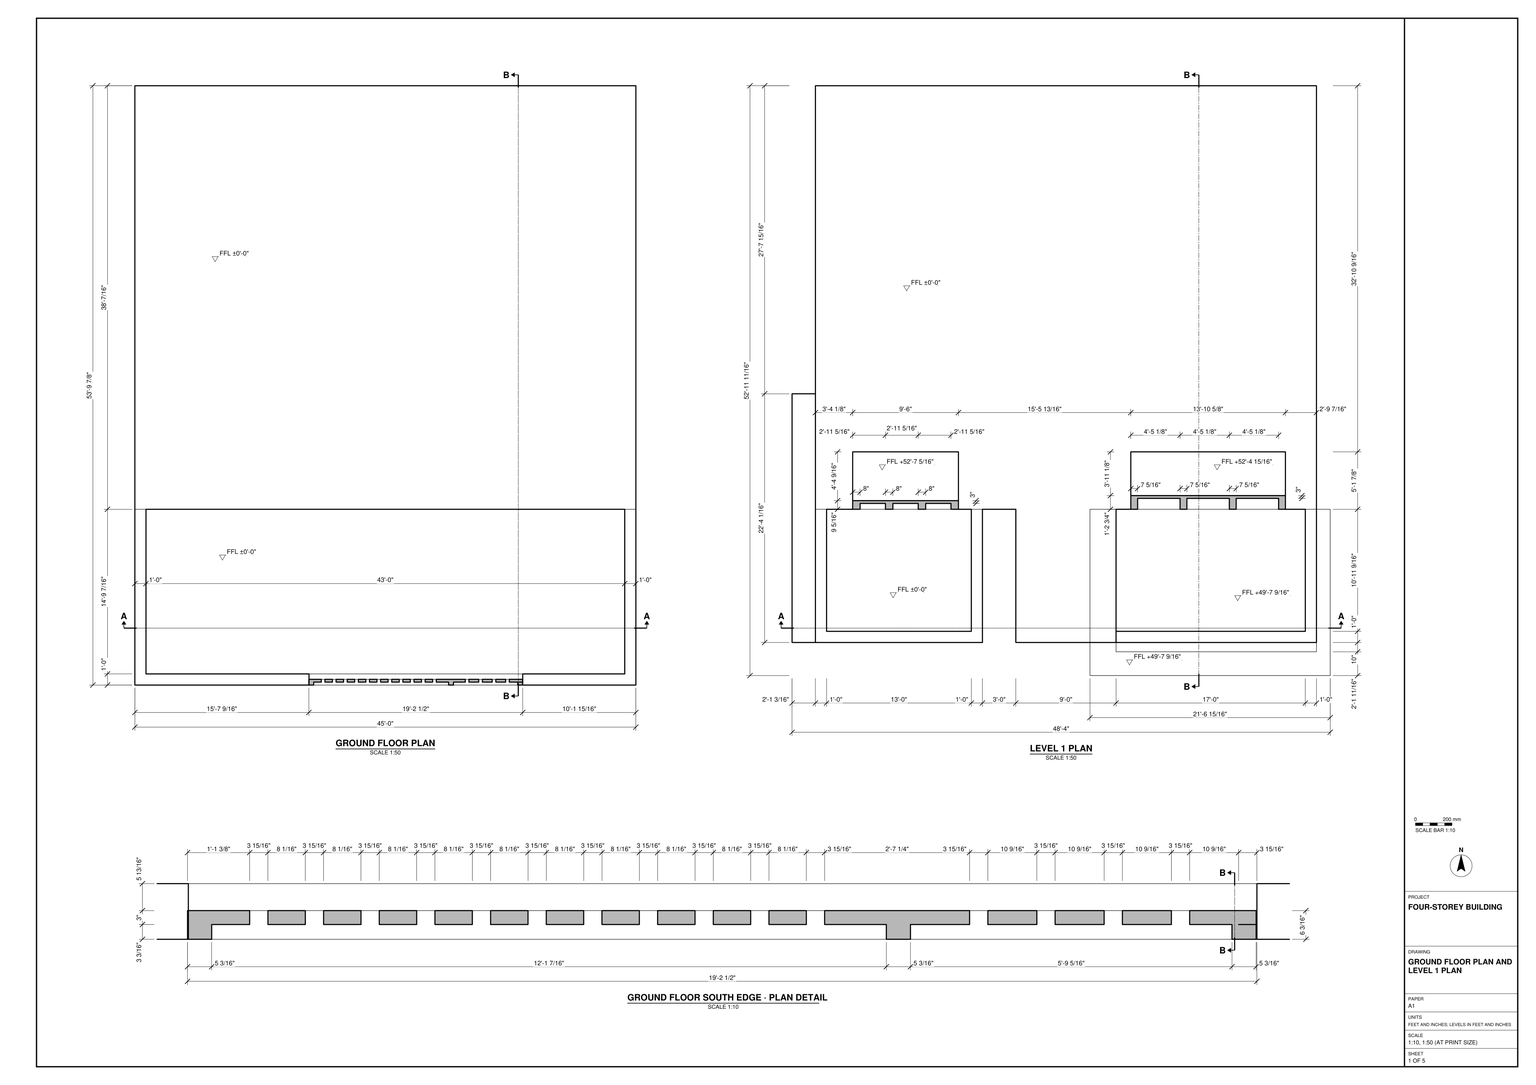
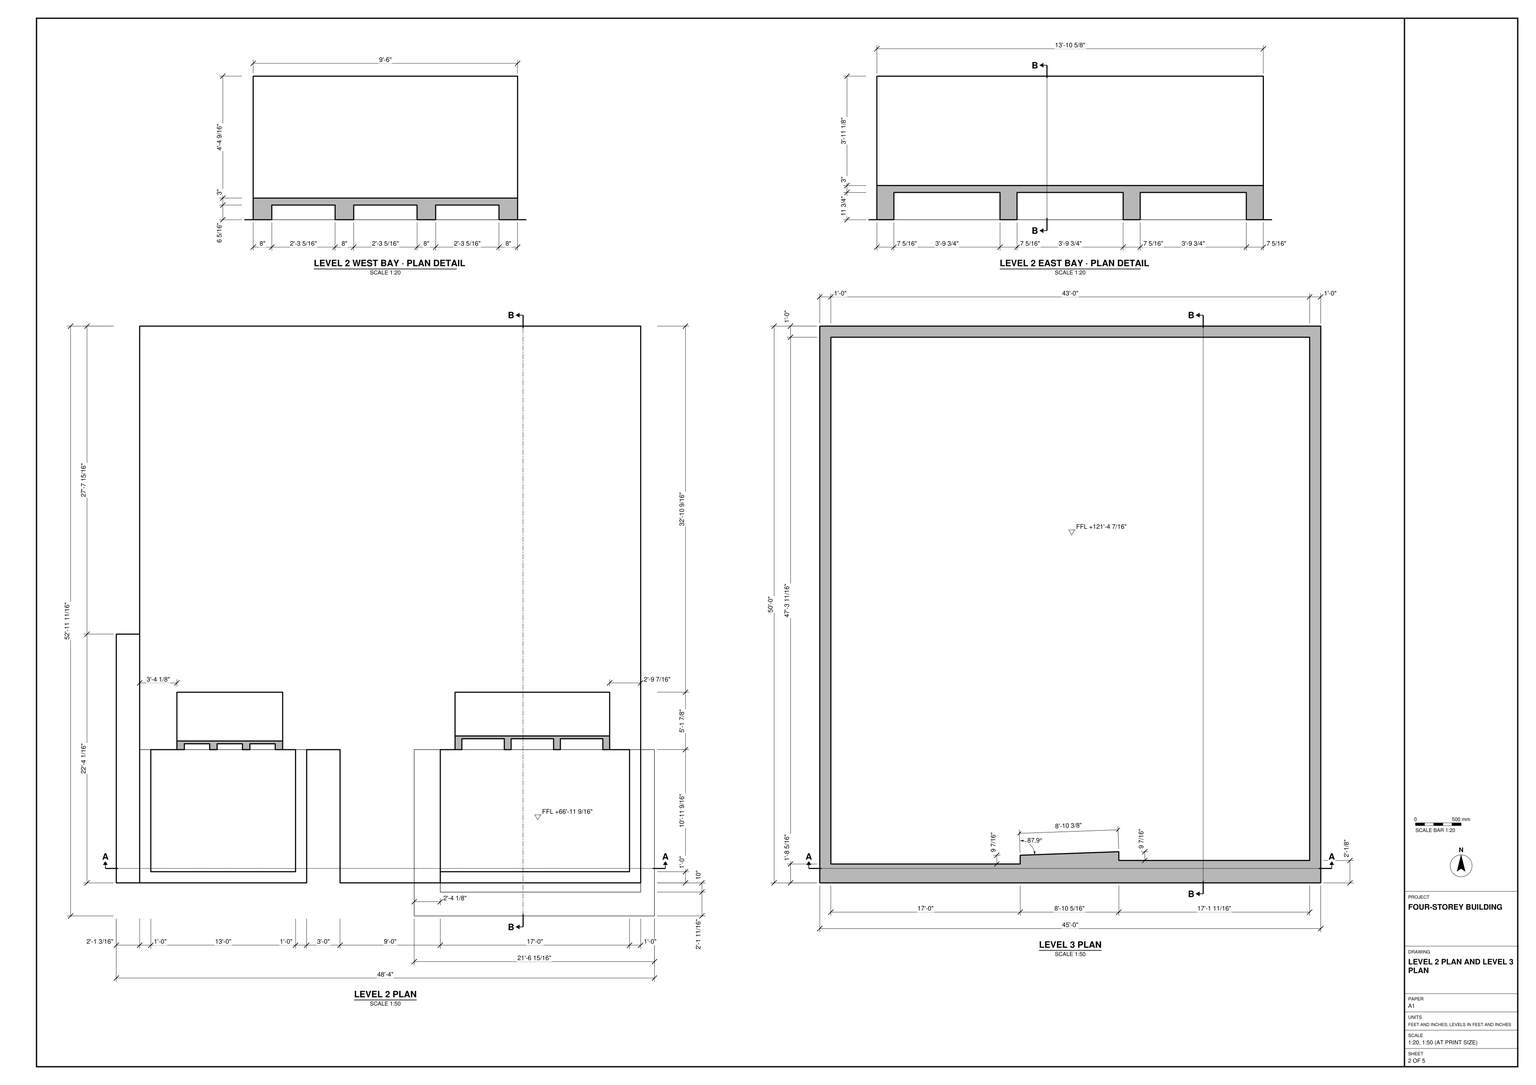
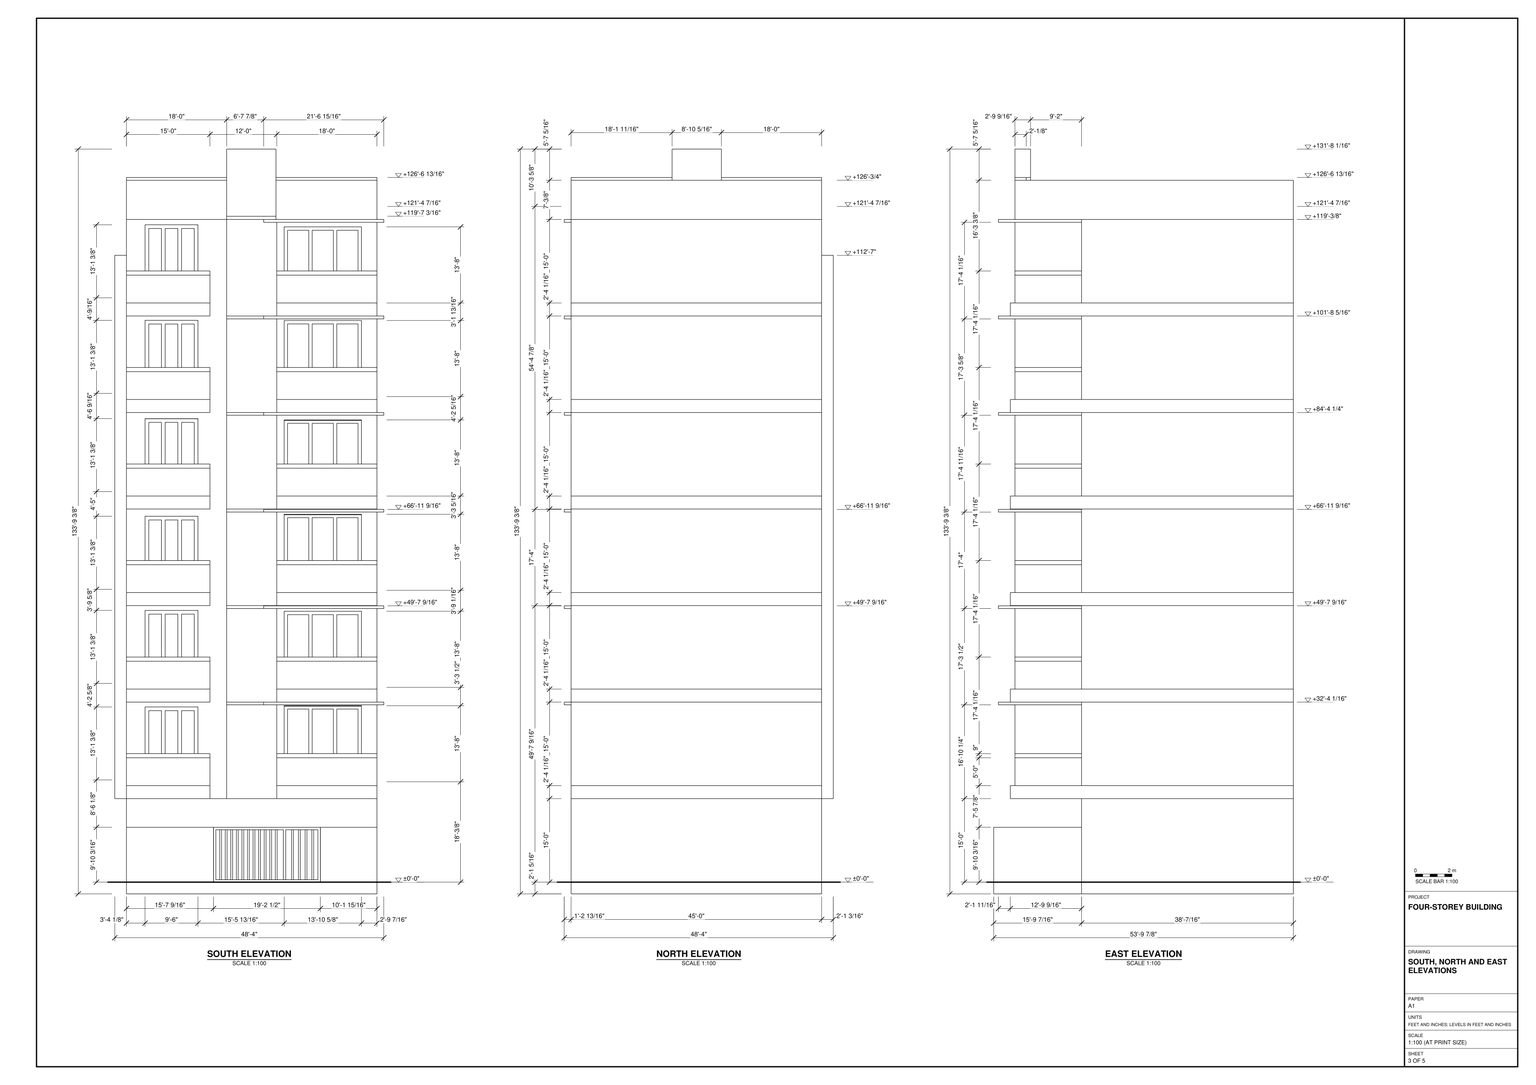
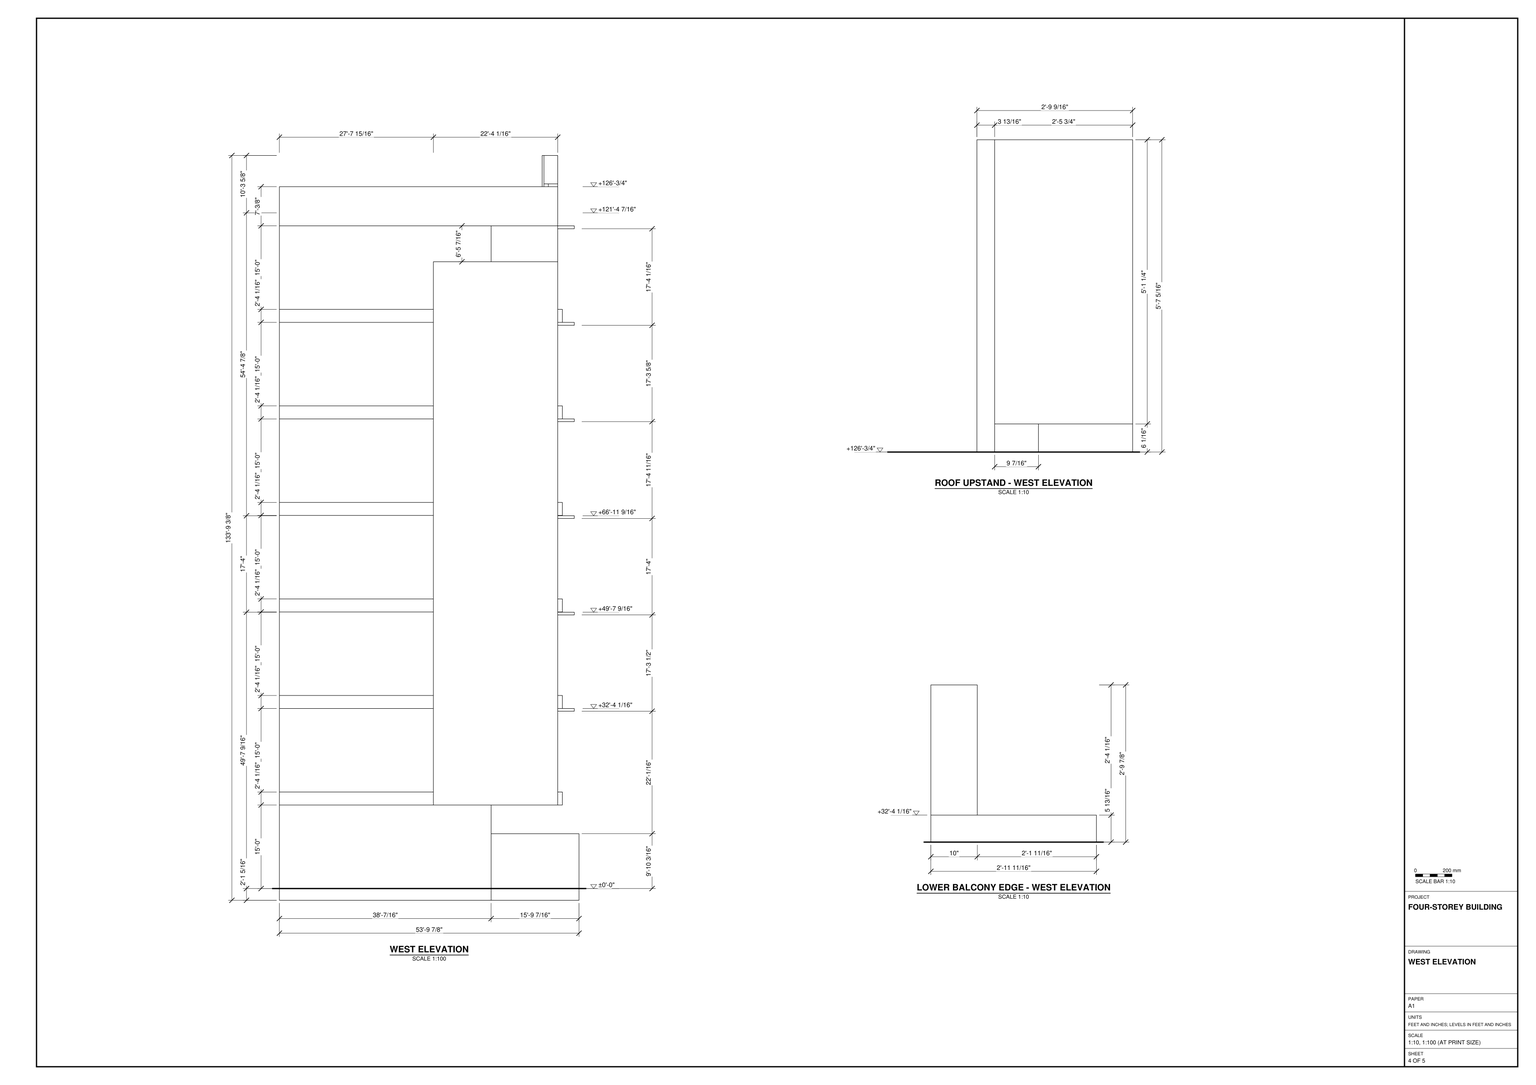
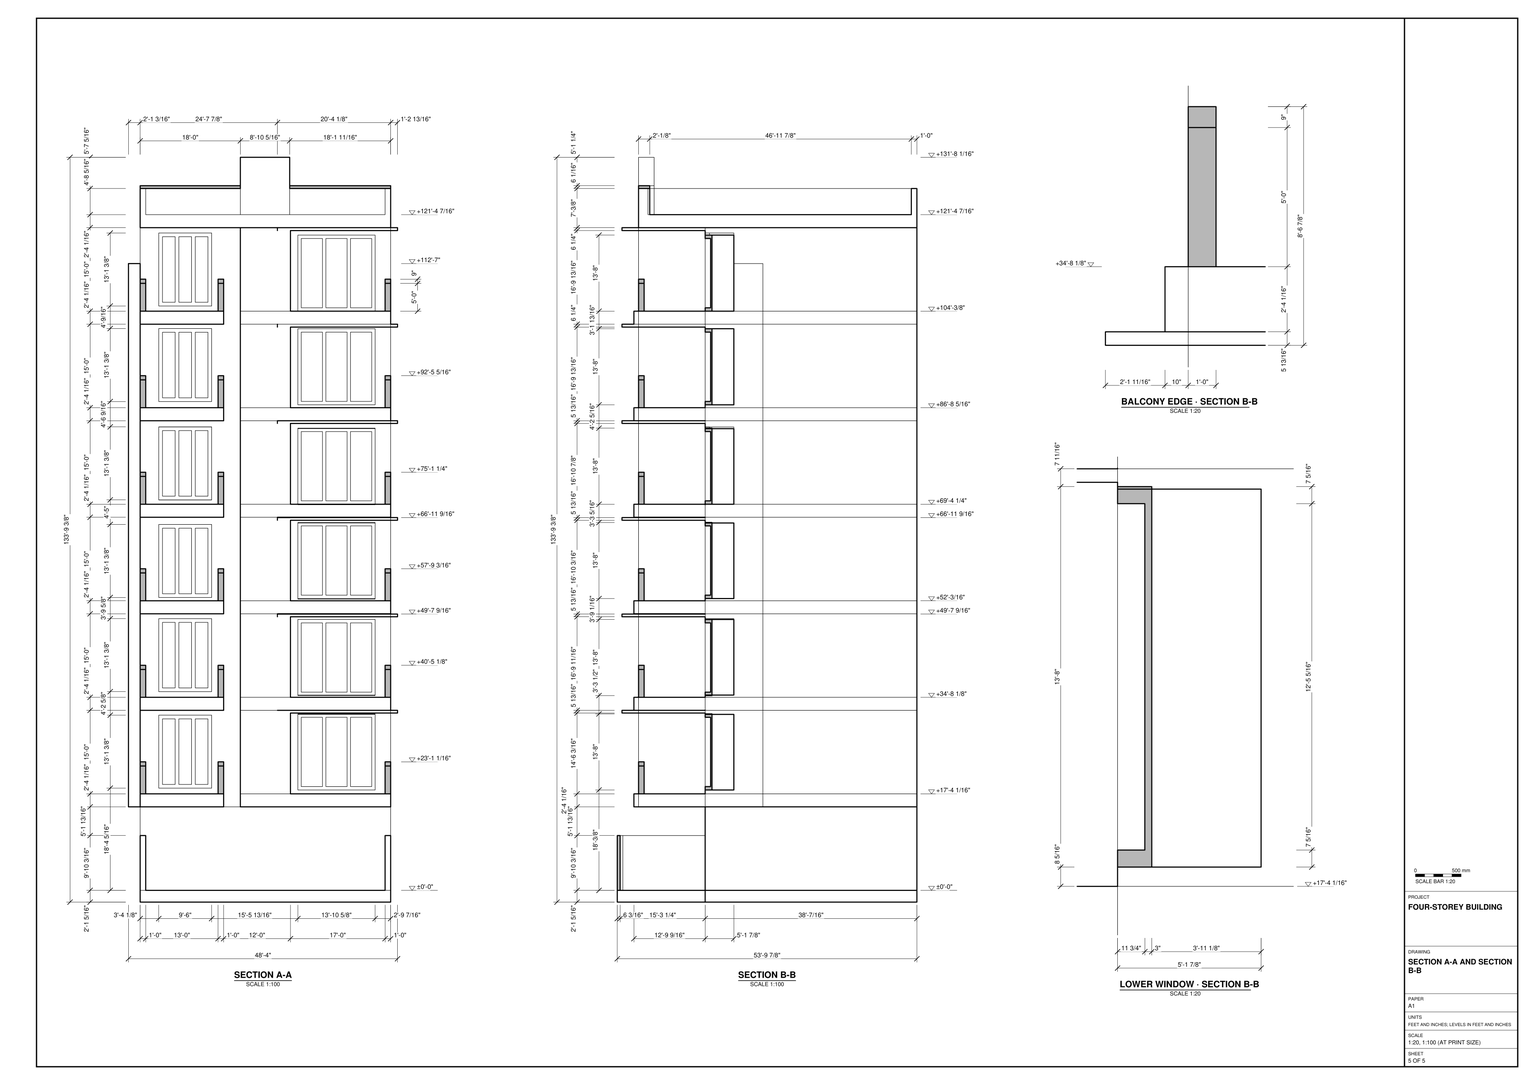
Build the four-storey building in SketchUp from task_files/diagram_01.pdf. Work in feet and inches. Set the overall width to 48'-4", depth to 53'-9 7/8" and height to 133'-9 3/8", including the projections. Use the floor levels ±0'-0", +49'-7 9/16", +66'-11 9/16" and +121'-4 7/16" relative to the ground floor.

Start with the rectangular ground-floor plan. Along its south edge, form the offset screen with closely spaced vertical members and solid wall to either side. Above it, build the narrower west bay and wider east bay with the setback between them. Use the plan details for the depth of the wall returns and the spacing of the framed openings. Follow the south elevation for all six tiers of openings, their solid lower fronts and the projecting slab edges. Keep the broad north face plain apart from the horizontal divisions shown. Finish the flat roof with its perimeter wall and the short raised section at the south edge.

Give walls and slabs their drawn thicknesses. Keep walls, slabs and roof elements in separate groups or components, group each furniture or joinery piece separately where shown, and use components for repeated parts. Any decor or loose items shown may use suitable library components. Save one SketchUp model as output_files/four_storey_building_with_stacked_south_facing_bays.skp.

# SketchUp Ruby script. Lengths in inches.
U = 1.inch
M = Sketchup.active_model
def pt(a) = Geom::Point3d.new(a.map { |v| v * U })
def face(e, loops, mat)
  f = e.add_face(loops[0].map { |a| pt(a) })
  loops[1..].each { |l| e.add_face(l.map { |a| pt(a) }).erase! }
  f.material = f.back_material = mat if mat
  f
end
# faces: each face lists its corners as indices into pts; further lists are holes
def faces(e, pts, list, mat = nil) = list.each { |f| face(e, (f[0].is_a?(Array) ? f : [f]).map { |l| l.map { |i| pts[i] } }, mat) }
# xy, xz, yz: faces in a plane at the given z, y or x. An outline is a flat list of corners, or four numbers for a rectangle; further outlines are holes
def ring(l) = l.size == 4 ? [[l[0], l[1]], [l[2], l[1]], [l[2], l[3]], [l[0], l[3]]] : l.each_slice(2).to_a
def flat(e, list, mat, &to3) = list.each { |f| face(e, (f[0].is_a?(Array) ? f : [f]).map { |l| ring(l).map { |u, v| to3.(u, v) } }, mat) }
def xy(e, z, list, mat = nil) = flat(e, list, mat) { |x, y| [x, y, z] }
def xz(e, y, list, mat = nil) = flat(e, list, mat) { |x, z| [x, y, z] }
def yz(e, x, list, mat = nil) = flat(e, list, mat) { |y, z| [x, y, z] }
def lines(e, pts, list) = list.each { |a, b| e.add_line(pt(pts[a]), pt(pts[b])) }
# prism: a flat outline (further loops are holes) pulled along v
def prism(e, loops, v, mat = nil)
  f = face(e, loops, mat); d = Geom::Vector3d.new(v.map { |x| x * U })
  f.pushpull(f.normal.samedirection?(d) ? d.length : -d.length)
end
def box(e, o, s, mat = nil) = prism(e, [[o, [o[0] + s[0], o[1], o[2]], [o[0] + s[0], o[1] + s[1], o[2]], [o[0], o[1] + s[1], o[2]]]], [0, 0, s[2]], mat)
def at(x, y, z, deg = 0) = Geom::Transformation.translation(pt([x, y, z])) * Geom::Transformation.rotation(ORIGIN, Z_AXIS, deg.degrees)
def axes(o, x, y, z) = Geom::Transformation.new([*x, 0, *y, 0, *z, 0, *pt(o).to_a, 1])
def part(name) = M.definitions.add(name)
# library, detail: a bought-in or finely detailed component or shape, given as its bounding box
def library(name, o, s) = part(name).tap { |d| box(d.entities, o, s) }
def detail(e, o, s) = box(e.add_group.entities, o, s)
def put(e, d, t, mat = nil) = e.add_instance(d, t).tap { |i| i.material = mat if mat }
def group(e, t, mat = nil) = e.add_group.tap { |g| g.transformation = t; g.material = mat if mat }.entities
root = M.entities
M.materials.add("[Brick Antique 01]").color = [173, 79, 62]
M.materials.add("[Color M07]").color = [58, 58, 58]
M.materials.add("[Color M08]").color = [30, 30, 30]
M.materials.add("[Translucent Glass Blue]").color = [98, 147, 234]
M.materials["[Translucent Glass Blue]"].alpha = 0.66
M.materials.add("[Translucent Glass Gray]").color = [128, 128, 128]
M.materials["[Translucent Glass Gray]"].alpha = 0.5
c1 = part("Group\#1")
xy(c1.entities,0,[[0,0,166.625,14.75]])
xy(c1.entities,7.34,[[7.34,0,53.1,11.75],[60.43,0,106.19,11.75],[113.53,0,159.29,11.75]])
xy(c1.entities,156.66,[[7.34,0,53.1,11.75],[60.43,0,106.19,11.75],[113.53,0,159.29,11.75]])
xy(c1.entities,164,[[0,0,166.625,14.75]])
xz(c1.entities,0,[[[0,0,166.625,164],[7.34,7.34,53.1,156.66],[60.43,7.34,106.19,156.66],[113.53,7.34,159.29,156.66]]])
xz(c1.entities,11.75,[[7.34,7.34,53.1,156.66],[60.43,7.34,106.19,156.66],[113.53,7.34,159.29,156.66]],"[Translucent Glass Gray]")
xz(c1.entities,14.75,[[0,0,166.625,164]],"[Translucent Glass Gray]")
yz(c1.entities,0,[[0,0,14.75,164]])
yz(c1.entities,7.34,[[0,7.34,11.75,156.66]])
yz(c1.entities,53.1,[[0,7.34,11.75,156.66]])
yz(c1.entities,60.43,[[0,7.34,11.75,156.66]])
yz(c1.entities,106.19,[[0,7.34,11.75,156.66]])
yz(c1.entities,113.53,[[0,7.34,11.75,156.66]])
yz(c1.entities,159.29,[[0,7.34,11.75,156.66]])
yz(c1.entities,166.625,[[0,0,14.75,164]])
c2 = part("Group\#2")
xy(c2.entities,0,[[0,0,114,9.3125]])
xy(c2.entities,8.02,[[8.02,0,35.33,6.3125],[43.35,0,70.65,6.3125],[78.67,0,105.98,6.3125]])
xy(c2.entities,149.35,[[8.02,0,35.33,6.3125],[43.35,0,70.65,6.3125],[78.67,0,105.98,6.3125]])
xy(c2.entities,157.375,[[0,0,114,9.3125]])
xz(c2.entities,0,[[[0,0,114,157.375],[78.67,8.02,105.98,149.35],[43.35,8.02,70.65,149.35],[8.02,8.02,35.33,149.35]]])
xz(c2.entities,6.3125,[[8.02,8.02,35.33,149.35],[43.35,8.02,70.65,149.35],[78.67,8.02,105.98,149.35]],"[Translucent Glass Gray]")
xz(c2.entities,9.3125,[[0,0,114,157.375]],"[Translucent Glass Gray]")
yz(c2.entities,0,[[0,0,9.3125,157.375]])
yz(c2.entities,8.02,[[0,8.02,6.3125,149.35]])
yz(c2.entities,35.33,[[0,8.02,6.3125,149.35]])
yz(c2.entities,43.35,[[0,8.02,6.3125,149.35]])
yz(c2.entities,70.65,[[0,8.02,6.3125,149.35]])
yz(c2.entities,78.67,[[0,8.02,6.3125,149.35]])
yz(c2.entities,105.98,[[0,8.02,6.3125,149.35]])
yz(c2.entities,114,[[0,0,9.3125,157.375]])
xy(root,-25.3125,[[25.1875,0,565.1875,189.4375],[25.1875,189.4375,565.1875,645.875]])
xy(root,0,[[212.91,0,443.25,12],[37.1875,12,553.1875,189.4375],[25.1875,189.4375,565.1875,645.875]])
xy(root,118.1875,[[25.1875,0,212.91,0,212.91,12,37.1875,12,37.1875,189.4375,25.1875,189.4375],[443.25,0,565.1875,0,565.1875,189.4375,553.1875,189.4375,553.1875,12,443.25,12]])
xy(root,180,[[349.1875,35.875,349.1875,45.875,241.1875,45.875,241.1875,189.4375,565.1875,189.4375,565.1875,35.875],[0,45.875,25.1875,313.91],[25.1875,45.875,205.1875,189.4375],[25.1875,189.4375,565.1875,645.875]])
xy(root,208.0625,[[349.1875,35.875,565.1875,45.875],[25.1875,45.875,25.1875,189.4375,37.1875,189.4375,37.1875,57.875,193.1875,57.875,193.1875,189.4375,205.1875,189.4375,205.1875,45.875],[349.1875,45.875,349.1875,57.875,553.1875,57.875,553.1875,189.4375,565.1875,189.4375,565.1875,45.875],[37.1875,57.875,193.1875,189.4375],[349.1875,57.875,553.1875,189.4375]])
xy(root,216.375,[[365.1,189.4375,531.73,251.3125]])
xy(root,220.3,[[65.3125,189.4375,179.3125,251.3125]])
xy(root,268.0625,[[25.1875,45.875,25.1875,189.4375,37.1875,189.4375,37.1875,57.875,193.1875,57.875,193.1875,189.4375,205.1875,189.4375,205.1875,45.875],[349.1875,45.875,349.1875,57.875,553.1875,57.875,553.1875,189.4375,565.1875,189.4375,565.1875,45.875]])
xy(root,277.0625,[[25.1875,45.875,205.1875,45.875,205.1875,189.4375,193.1875,189.4375,193.1875,57.875,37.1875,57.875,37.1875,189.4375,25.1875,189.4375],[349.1875,45.875,565.1875,45.875,565.1875,189.4375,553.1875,189.4375,553.1875,57.875,349.1875,57.875]])
xy(root,377.67,[[65.3125,189.4375,179.3125,251.3125]])
xy(root,379.3125,[[365.1,189.4375,531.73,251.3125]])
xy(root,382.25,[[321.0625,10.1875,321.0625,45.875,349.1875,45.875,349.1875,189.4375,580,189.4375,580,10.1875]])
xy(root,388.0625,[[321.0625,10.1875,565.1875,10.1875,565.1875,35.875,349.1875,35.875,349.1875,45.875,321.0625,45.875],[565.1875,10.1875,580,189.4375],[349.1875,35.875,349.1875,45.875,321.0625,45.875,321.0625,189.4375,565.1875,189.4375,565.1875,35.875],[25.1875,45.875,205.1875,189.4375]])
xy(root,416.125,[[349.1875,35.875,565.1875,45.875],[25.1875,45.875,25.1875,189.4375,37.1875,189.4375,37.1875,57.875,193.1875,57.875,193.1875,189.4375,205.1875,189.4375,205.1875,45.875],[349.1875,45.875,349.1875,57.875,553.1875,57.875,553.1875,189.4375,565.1875,189.4375,565.1875,45.875],[37.1875,57.875,193.1875,189.4375],[349.1875,57.875,553.1875,189.4375]])
xy(root,420.9375,[[365.1,189.4375,531.73,251.3125]])
xy(root,428.3,[[65.3125,189.4375,179.3125,251.3125]])
xy(root,476.125,[[25.1875,45.875,25.1875,189.4375,37.1875,189.4375,37.1875,57.875,193.1875,57.875,193.1875,189.4375,205.1875,189.4375,205.1875,45.875],[349.1875,45.875,349.1875,57.875,553.1875,57.875,553.1875,189.4375,565.1875,189.4375,565.1875,45.875]])
xy(root,485.125,[[25.1875,45.875,205.1875,45.875,205.1875,189.4375,193.1875,189.4375,193.1875,57.875,37.1875,57.875,37.1875,189.4375,25.1875,189.4375],[349.1875,45.875,565.1875,45.875,565.1875,189.4375,553.1875,189.4375,553.1875,57.875,349.1875,57.875]])
xy(root,583.875,[[365.1,189.4375,531.73,251.3125]])
xy(root,585.67,[[65.3125,189.4375,179.3125,251.3125]])
xy(root,589.72,[[321.0625,10.1875,321.0625,45.875,349.1875,45.875,349.1875,189.4375,580,189.4375,580,10.1875]])
xy(root,595.53,[[321.0625,10.1875,580,189.4375]])
xy(root,596.125,[[349.1875,35.875,349.1875,45.875,321.0625,45.875,321.0625,189.4375,565.1875,189.4375,565.1875,35.875],[25.1875,45.875,205.1875,189.4375]])
xy(root,624.1875,[[349.1875,35.875,565.1875,45.875],[25.1875,45.875,25.1875,189.4375,37.1875,189.4375,37.1875,57.875,193.1875,57.875,193.1875,189.4375,205.1875,189.4375,205.1875,45.875],[349.1875,45.875,349.1875,57.875,553.1875,57.875,553.1875,189.4375,565.1875,189.4375,565.1875,45.875],[37.1875,57.875,193.1875,189.4375],[349.1875,57.875,553.1875,189.4375]])
xy(root,628.9375,[[365.1,189.4375,531.73,251.3125]])
xy(root,631.3,[[65.3125,189.4375,179.3125,251.3125]])
xy(root,684.1875,[[25.1875,45.875,25.1875,189.4375,37.1875,189.4375,37.1875,57.875,193.1875,57.875,193.1875,189.4375,205.1875,189.4375,205.1875,45.875],[349.1875,45.875,349.1875,57.875,553.1875,57.875,553.1875,189.4375,565.1875,189.4375,565.1875,45.875]])
xy(root,693.1875,[[25.1875,45.875,205.1875,45.875,205.1875,189.4375,193.1875,189.4375,193.1875,57.875,37.1875,57.875,37.1875,189.4375,25.1875,189.4375],[349.1875,45.875,565.1875,45.875,565.1875,189.4375,553.1875,189.4375,553.1875,57.875,349.1875,57.875]])
xy(root,788.67,[[65.3125,189.4375,179.3125,251.3125]])
xy(root,791.875,[[365.1,189.4375,531.73,251.3125]])
xy(root,797.72,[[321.0625,10.1875,321.0625,45.875,349.1875,45.875,349.1875,189.4375,580,189.4375,580,10.1875]])
xy(root,803.53,[[321.0625,10.1875,580,189.4375]])
xy(root,804.1875,[[349.1875,35.875,349.1875,45.875,321.0625,45.875,321.0625,189.4375,565.1875,189.4375,565.1875,35.875],[25.1875,45.875,205.1875,189.4375]])
xy(root,832.25,[[349.1875,35.875,565.1875,45.875],[25.1875,45.875,25.1875,189.4375,37.1875,189.4375,37.1875,57.875,193.1875,57.875,193.1875,189.4375,205.1875,189.4375,205.1875,45.875],[349.1875,45.875,349.1875,57.875,553.1875,57.875,553.1875,189.4375,565.1875,189.4375,565.1875,45.875],[37.1875,57.875,193.1875,189.4375],[349.1875,57.875,553.1875,189.4375],
  [365.1,189.4375,531.73,251.3125]])
xy(root,841.42,[[65.3125,189.4375,179.3125,251.3125]])
xy(root,892.25,[[25.1875,45.875,25.1875,189.4375,37.1875,189.4375,37.1875,57.875,193.1875,57.875,193.1875,189.4375,205.1875,189.4375,205.1875,45.875],[349.1875,45.875,349.1875,57.875,553.1875,57.875,553.1875,189.4375,565.1875,189.4375,565.1875,45.875]])
xy(root,901.25,[[25.1875,45.875,205.1875,45.875,205.1875,189.4375,193.1875,189.4375,193.1875,57.875,37.1875,57.875,37.1875,189.4375,25.1875,189.4375],[349.1875,45.875,565.1875,45.875,565.1875,189.4375,553.1875,189.4375,553.1875,57.875,349.1875,57.875]])
xy(root,995.1875,[[365.1,189.4375,531.73,251.3125]])
xy(root,998.8,[[65.3125,189.4375,179.3125,251.3125]])
xy(root,1006.4375,[[321.0625,10.1875,321.0625,45.875,349.1875,45.875,349.1875,189.4375,580,189.4375,580,10.1875]])
xy(root,1012.25,[[321.0625,10.1875,580,10.1875,580,189.4375,565.1875,189.4375,565.1875,35.875,349.1875,35.875,349.1875,45.875,321.0625,45.875],[349.1875,35.875,349.1875,45.875,321.0625,45.875,321.0625,189.4375,565.1875,189.4375,565.1875,35.875],[25.1875,45.875,205.1875,189.4375]])
xy(root,1040.3125,[[349.1875,35.875,565.1875,45.875],[25.1875,45.875,25.1875,189.4375,37.1875,189.4375,37.1875,57.875,193.1875,57.875,193.1875,189.4375,205.1875,189.4375,205.1875,45.875],[349.1875,45.875,349.1875,57.875,553.1875,57.875,553.1875,189.4375,565.1875,189.4375,565.1875,45.875],[37.1875,57.875,193.1875,189.4375],[349.1875,57.875,553.1875,189.4375]])
xy(root,1046.5625,[[365.1,189.4375,531.73,251.3125]])
xy(root,1053.61,[[65.3125,189.4375,179.3125,251.3125]])
xy(root,1100.3125,[[25.1875,45.875,25.1875,189.4375,37.1875,189.4375,37.1875,57.875,193.1875,57.875,193.1875,189.4375,205.1875,189.4375,205.1875,45.875],[349.1875,45.875,349.1875,57.875,553.1875,57.875,553.1875,189.4375,565.1875,189.4375,565.1875,45.875]])
xy(root,1109.3125,[[25.1875,45.875,205.1875,45.875,205.1875,189.4375,193.1875,189.4375,193.1875,57.875,37.1875,57.875,37.1875,189.4375,25.1875,189.4375],[349.1875,45.875,565.1875,45.875,565.1875,189.4375,553.1875,189.4375,553.1875,57.875,349.1875,57.875]])
xy(root,1210.5625,[[365.1,189.4375,531.73,251.3125]])
xy(root,1210.98,[[65.3125,189.4375,179.3125,251.3125]])
xy(root,1214.0625,[[321.0625,10.1875,321.0625,45.875,349.1875,45.875,349.1875,189.4375,580,189.4375,580,10.1875]])
xy(root,1220.3125,[[321.0625,10.1875,580,10.1875,580,189.4375,565.1875,189.4375,565.1875,35.875,349.1875,35.875,349.1875,45.875,321.0625,45.875],[25.1875,45.875,205.1875,189.4375]])
xy(root,1248.375,[[349.1875,35.875,565.1875,45.875],[25.1875,45.875,25.1875,189.4375,37.1875,189.4375,37.1875,57.875,193.1875,57.875,193.1875,189.4375,205.1875,189.4375,205.1875,45.875],[349.1875,45.875,349.1875,57.875,553.1875,57.875,553.1875,189.4375,565.1875,189.4375,565.1875,45.875],[37.1875,57.875,193.1875,189.4375],[349.1875,57.875,349.1875,189.4375,365.1,189.4375,365.1,251.3125,531.73,251.3125,531.73,189.4375,553.1875,189.4375,553.1875,57.875]])
xy(root,1259.55,[[65.3125,189.4375,179.3125,251.3125]])
xy(root,1308.375,[[25.1875,45.875,25.1875,189.4375,37.1875,189.4375,37.1875,57.875,193.1875,57.875,193.1875,189.4375,205.1875,189.4375,205.1875,45.875],[349.1875,45.875,349.1875,57.875,553.1875,57.875,553.1875,189.4375,565.1875,189.4375,565.1875,45.875]])
xy(root,1317.375,[[25.1875,45.875,205.1875,45.875,205.1875,189.4375,193.1875,189.4375,193.1875,57.875,37.1875,57.875,37.1875,189.4375,25.1875,189.4375],[349.1875,45.875,565.1875,45.875,565.1875,189.4375,553.1875,189.4375,553.1875,57.875,349.1875,57.875]])
xy(root,1351.03,[[0,45.875,25.1875,313.91]])
xy(root,1412.375,[[365.1,189.4375,531.73,251.3125]])
xy(root,1416.92,[[65.3125,189.4375,179.3125,251.3125]])
xy(root,1422.125,[[321.0625,10.1875,321.0625,45.875,349.1875,45.875,349.1875,189.4375,580,189.4375,580,10.1875]])
xy(root,1428.375,[[321.0625,10.1875,580,10.1875,580,189.4375,565.1875,189.4375,565.1875,45.875,321.0625,45.875],[241.1875,45.875,241.1875,189.4375,25.1875,189.4375,25.1875,645.875,565.1875,645.875,565.1875,45.875],[25.1875,45.875,241.1875,189.4375]])
xy(root,1456.4375,[[37.1875,66.1875,241.1875,66.1875,241.1875,75.625,347.52,79.45,347.52,70.01,553.1875,70.01,553.1875,633.875,37.1875,633.875]])
xy(root,1512.75,[[25.1875,45.875,241.1875,66.1875],[347.52,45.875,565.1875,70.01],[25.1875,66.1875,37.1875,66.1875,37.1875,633.875,553.1875,633.875,553.1875,70.01,565.1875,70.01,565.1875,645.875,25.1875,645.875]])
xy(root,1518.8125,[[25.1875,45.875,241.1875,66.1875],[347.52,45.875,565.1875,70.01]])
xy(root,1580.0625,[[241.1875,45.875,347.52,45.875,347.52,79.45,241.1875,75.625]])
xz(root,0,[[25.1875,-25.3125,565.1875,-25.3125,565.1875,118.1875,443.25,118.1875,443.25,0,212.91,0,212.91,118.1875,25.1875,118.1875]])
xz(root,10.1875,[[321.0625,382.25,580,388.0625],[321.0625,589.72,580,595.53],[321.0625,797.72,580,803.53],[321.0625,1006.4375,580,1012.25],[321.0625,1214.0625,580,1220.3125],
  [321.0625,1422.125,580,1428.375]])
xz(root,12,[[37.1875,0,212.91,118.1875],[443.25,0,553.1875,118.1875]])
xz(root,35.875,[[349.1875,180,565.1875,208.0625],[349.1875,388.0625,565.1875,416.125],[349.1875,596.125,565.1875,624.1875],[349.1875,804.1875,565.1875,832.25],[349.1875,1012.25,565.1875,1040.3125],
  [349.1875,1220.3125,565.1875,1248.375]])
xz(root,45.875,[[0,180,25.1875,1351.03],[25.1875,180,205.1875,208.0625],[25.1875,268.0625,205.1875,277.0625],[349.1875,268.0625,565.1875,277.0625],[241.1875,382.25,321.0625,388.0625],
  [25.1875,388.0625,205.1875,416.125],[25.1875,476.125,205.1875,485.125],[349.1875,476.125,565.1875,485.125],[241.1875,589.72,321.0625,596.125],[25.1875,596.125,205.1875,624.1875],
  [25.1875,684.1875,205.1875,693.1875],[349.1875,684.1875,565.1875,693.1875],[241.1875,797.72,321.0625,804.1875],[25.1875,804.1875,205.1875,832.25],[25.1875,892.25,205.1875,901.25],
  [349.1875,892.25,565.1875,901.25],[241.1875,1006.4375,321.0625,1012.25],[25.1875,1012.25,205.1875,1040.3125],[25.1875,1100.3125,205.1875,1109.3125],[349.1875,1100.3125,565.1875,1109.3125],
  [241.1875,1214.0625,321.0625,1220.3125],[25.1875,1220.3125,205.1875,1248.375],[25.1875,1308.375,205.1875,1317.375],[349.1875,1308.375,565.1875,1317.375],[241.1875,1428.375,347.52,1435.1875],
  [25.1875,1512.75,241.1875,1518.8125],[347.52,1512.75,565.1875,1518.8125]])
xz(root,45.875,[[241.1875,180,349.1875,382.25],[241.1875,388.0625,349.1875,589.72],[241.1875,596.125,349.1875,797.72],[241.1875,804.1875,349.1875,1006.4375],[241.1875,1012.25,349.1875,1214.0625],
  [241.1875,1220.3125,349.1875,1220.3125,349.1875,1422.125,321.0625,1422.125,321.0625,1428.375,241.1875,1428.375],[241.1875,1435.1875,347.52,1580.0625]],"[Brick Antique 01]")
xz(root,45.875,[[25.1875,208.0625,205.1875,268.0625],[25.1875,416.125,205.1875,476.125],[25.1875,624.1875,205.1875,684.1875],[25.1875,832.25,205.1875,892.25],[25.1875,1040.3125,205.1875,1100.3125],
  [25.1875,1248.375,205.1875,1308.375]],"[Translucent Glass Blue]")
xz(root,45.875,[[349.1875,208.0625,565.1875,268.0625],[349.1875,416.125,565.1875,476.125],[349.1875,624.1875,565.1875,684.1875],[349.1875,832.25,565.1875,892.25],[349.1875,1040.3125,565.1875,1100.3125],
  [349.1875,1248.375,565.1875,1308.375],[25.1875,1428.375,241.1875,1512.75],[347.52,1428.375,565.1875,1512.75]],"[Translucent Glass Gray]")
xz(root,57.875,[[37.1875,268.0625,193.1875,277.0625],[349.1875,268.0625,553.1875,277.0625],[37.1875,476.125,193.1875,485.125],[349.1875,476.125,553.1875,485.125],[37.1875,684.1875,193.1875,693.1875],
  [349.1875,684.1875,553.1875,693.1875],[37.1875,892.25,193.1875,901.25],[349.1875,892.25,553.1875,901.25],[37.1875,1100.3125,193.1875,1109.3125],[349.1875,1100.3125,553.1875,1109.3125],
  [37.1875,1308.375,193.1875,1317.375],[349.1875,1308.375,553.1875,1317.375]])
xz(root,57.875,[[37.1875,208.0625,193.1875,268.0625],[349.1875,208.0625,553.1875,268.0625],[37.1875,416.125,193.1875,476.125],[349.1875,416.125,553.1875,476.125],[37.1875,624.1875,193.1875,684.1875],
  [349.1875,624.1875,553.1875,684.1875],[37.1875,832.25,193.1875,892.25],[349.1875,832.25,553.1875,892.25],[37.1875,1040.3125,193.1875,1100.3125],[349.1875,1040.3125,553.1875,1100.3125],
  [37.1875,1248.375,193.1875,1308.375],[349.1875,1248.375,553.1875,1308.375]],"[Translucent Glass Gray]")
xz(root,66.1875,[[25.1875,1512.75,241.1875,1518.8125]])
xz(root,66.1875,[[37.1875,1456.4375,241.1875,1512.75]],"[Translucent Glass Gray]")
xz(root,70.01,[[347.52,1512.75,565.1875,1518.8125]])
xz(root,70.01,[[347.52,1456.4375,553.1875,1512.75]],"[Translucent Glass Gray]")
xz(root,189.4375,[[25.1875,-25.3125,565.1875,0],[37.1875,0,553.1875,0,553.1875,118.1875,565.1875,118.1875,565.1875,180,25.1875,180,25.1875,118.1875,37.1875,118.1875],[[205.1875,180,241.1875,180,241.1875,1428.375,25.1875,1428.375,25.1875,1317.375,37.1875,1317.375,37.1875,1248.375,193.1875,1248.375,193.1875,1317.375,205.1875,1317.375,205.1875,1220.3125,25.1875,1220.3125,25.1875,1109.3125,37.1875,1109.3125,37.1875,1040.3125,193.1875,1040.3125,193.1875,1109.3125,205.1875,1109.3125,205.1875,1012.25,25.1875,1012.25,25.1875,901.25,37.1875,901.25,37.1875,832.25,193.1875,832.25,193.1875,901.25,205.1875,901.25,205.1875,804.1875,25.1875,804.1875,25.1875,693.1875,37.1875,693.1875,37.1875,624.1875,193.1875,624.1875,193.1875,693.1875,205.1875,693.1875,205.1875,596.125,25.1875,596.125,25.1875,485.125,37.1875,485.125,37.1875,416.125,193.1875,416.125,193.1875,485.125,205.1875,485.125,205.1875,388.0625,25.1875,388.0625,25.1875,277.0625,37.1875,277.0625,37.1875,208.0625,193.1875,208.0625,193.1875,277.0625,205.1875,277.0625],[65.3125,1259.55,179.3125,1416.92],[65.3125,841.42,179.3125,998.8],[65.3125,631.3,179.3125,788.67],[65.3125,428.3,179.3125,585.67],[65.3125,220.3,179.3125,377.67],[65.3125,1053.61,179.3125,1210.98]],[[349.1875,208.0625,553.1875,208.0625,553.1875,277.0625,565.1875,277.0625,565.1875,382.25,349.1875,382.25],[365.1,216.375,531.73,379.3125]],[565.1875,382.25,580,388.0625],
  [366.76,388.0625,535.2,388.5],[[349.1875,416.125,553.1875,416.125,553.1875,485.125,565.1875,485.125,565.1875,589.72,349.1875,589.72],[365.1,419.875,531.73,583.875]],[365.1,419.875,531.73,420.9375],[565.1875,589.72,580,595.53],[321.0625,595.53,366.76,595.53,366.76,595.97,535.2,595.97,535.2,595.53,565.1875,595.53,565.1875,596.125,321.0625,596.125],
  [366.76,595.53,535.2,595.97],[[349.1875,624.1875,553.1875,624.1875,553.1875,693.1875,565.1875,693.1875,565.1875,797.72,349.1875,797.72],[365.1,627.875,531.73,791.875]],[365.1,627.875,531.73,628.9375],[565.1875,797.72,580,803.53],[321.0625,803.53,366.76,803.53,366.76,803.97,535.2,803.97,535.2,803.53,565.1875,803.53,565.1875,804.1875,321.0625,804.1875],
  [366.76,803.53,535.2,803.97],[365.1,831.1875,531.73,832.25],[349.1875,832.25,365.1,832.25,365.1,995.1875,531.73,995.1875,531.73,832.25,553.1875,832.25,553.1875,901.25,565.1875,901.25,565.1875,1006.4375,349.1875,1006.4375],[565.1875,1006.4375,580,1012.25],[366.76,1012.25,535.2,1012.6875],
  [[349.1875,1040.3125,553.1875,1040.3125,553.1875,1109.3125,565.1875,1109.3125,565.1875,1214.0625,349.1875,1214.0625],[365.1,1046.5625,531.73,1210.5625]],[565.1875,1214.0625,580,1220.3125],[25.1875,1248.375,37.1875,1308.375],[349.1875,1248.375,365.1,1248.375,365.1,1412.375,531.73,1412.375,531.73,1248.375,553.1875,1248.375,553.1875,1317.375,565.1875,1317.375,565.1875,1422.125,349.1875,1422.125],[25.1875,1308.375,37.1875,1317.375],
  [565.1875,1422.125,580,1428.375]])
xz(root,251.3125,[[365.1,216.375,531.73,379.3125],[65.3125,220.3,179.3125,377.67],[365.1,420.9375,531.73,583.875],[65.3125,428.3,179.3125,585.67],[365.1,628.9375,531.73,791.875],
  [65.3125,631.3,179.3125,788.67],[365.1,832.25,531.73,995.1875],[65.3125,841.42,179.3125,998.8],[365.1,1046.5625,531.73,1210.5625],[65.3125,1053.61,179.3125,1210.98],
  [365.1,1248.375,531.73,1412.375],[65.3125,1259.55,179.3125,1416.92]])
xz(root,313.91,[[0,180,25.1875,1351.03]])
xz(root,633.875,[[37.1875,1456.4375,553.1875,1512.75]])
xz(root,645.875,[[25.1875,-25.3125,565.1875,0],[25.1875,0,565.1875,180],[25.1875,180,565.1875,208.0625],[25.1875,208.0625,565.1875,388.0625],[25.1875,388.0625,565.1875,416.125],
  [25.1875,416.125,565.1875,596.125],[25.1875,596.125,565.1875,624.1875],[25.1875,624.1875,565.1875,804.1875],[25.1875,804.1875,565.1875,832.25],[25.1875,832.25,565.1875,1012.25],
  [25.1875,1012.25,565.1875,1040.3125],[25.1875,1040.3125,565.1875,1220.3125],[25.1875,1220.3125,565.1875,1248.375],[25.1875,1248.375,565.1875,1428.375],[25.1875,1428.375,565.1875,1512.75]])
yz(root,0,[[45.875,180,313.91,1351.03]])
yz(root,25.1875,[[0,-25.3125,189.4375,118.1875],[189.4375,-25.3125,645.875,0],[189.4375,0,645.875,180],[45.875,180,189.4375,208.0625],[189.4375,180,313.91,208.0625],
  [313.91,180,645.875,208.0625],[189.4375,208.0625,313.91,388.0625],[313.91,208.0625,645.875,388.0625],[45.875,268.0625,189.4375,277.0625],[45.875,277.0625,189.4375,388.0625],
  [45.875,388.0625,189.4375,416.125],[189.4375,388.0625,313.91,416.125],[313.91,388.0625,645.875,416.125],[189.4375,416.125,313.91,596.125],[313.91,416.125,645.875,596.125],
  [45.875,476.125,189.4375,485.125],[45.875,485.125,189.4375,596.125],[45.875,596.125,189.4375,624.1875],[189.4375,596.125,313.91,624.1875],[313.91,596.125,645.875,624.1875],
  [189.4375,624.1875,313.91,804.1875],[313.91,624.1875,645.875,804.1875],[45.875,684.1875,189.4375,693.1875],[45.875,693.1875,189.4375,804.1875],[45.875,804.1875,189.4375,832.25],
  [189.4375,804.1875,313.91,832.25],[313.91,804.1875,645.875,832.25],[189.4375,832.25,313.91,1012.25],[313.91,832.25,645.875,1012.25],[45.875,892.25,189.4375,901.25],
  [45.875,901.25,189.4375,1012.25],[45.875,1012.25,189.4375,1040.3125],[189.4375,1012.25,313.91,1040.3125],[313.91,1012.25,645.875,1040.3125],[189.4375,1040.3125,313.91,1220.3125],
  [313.91,1040.3125,645.875,1220.3125],[45.875,1100.3125,189.4375,1109.3125],[45.875,1109.3125,189.4375,1220.3125],[45.875,1220.3125,189.4375,1248.375],[189.4375,1220.3125,313.91,1248.375],
  [313.91,1220.3125,645.875,1248.375],[45.875,1248.375,189.4375,1308.375],[189.4375,1248.375,313.91,1351.03],[313.91,1248.375,313.91,1351.03,189.4375,1351.03,189.4375,1428.375,645.875,1428.375,645.875,1248.375],[45.875,1308.375,189.4375,1317.375],
  [45.875,1317.375,189.4375,1351.03],[45.875,1428.375,645.875,1512.75],[45.875,1512.75,66.1875,1518.8125]])
yz(root,25.1875,[[45.875,208.0625,189.4375,268.0625],[45.875,416.125,189.4375,476.125],[45.875,624.1875,189.4375,684.1875],[45.875,832.25,189.4375,892.25],[45.875,1040.3125,189.4375,1100.3125]],"[Translucent Glass Gray]")
yz(root,37.1875,[[12,0,189.4375,118.1875],[57.875,268.0625,189.4375,277.0625],[57.875,476.125,189.4375,485.125],[57.875,684.1875,189.4375,693.1875],[57.875,892.25,189.4375,901.25],
  [57.875,1100.3125,189.4375,1109.3125],[57.875,1308.375,189.4375,1317.375],[66.1875,1456.4375,633.875,1512.75]])
yz(root,37.1875,[[57.875,208.0625,189.4375,268.0625],[57.875,416.125,189.4375,476.125],[57.875,624.1875,189.4375,684.1875],[57.875,832.25,189.4375,892.25],[57.875,1040.3125,189.4375,1100.3125],
  [57.875,1248.375,189.4375,1308.375]],"[Translucent Glass Gray]")
yz(root,65.3125,[[189.4375,220.3,251.3125,377.67],[189.4375,428.3,251.3125,585.67],[189.4375,631.3,251.3125,788.67],[189.4375,841.42,251.3125,998.8],[189.4375,1053.61,251.3125,1210.98],
  [189.4375,1259.55,251.3125,1416.92]])
yz(root,179.3125,[[189.4375,220.3,251.3125,377.67],[189.4375,428.3,251.3125,585.67],[189.4375,631.3,251.3125,788.67],[189.4375,841.42,251.3125,998.8],[189.4375,1053.61,251.3125,1210.98],
  [189.4375,1259.55,251.3125,1416.92]])
yz(root,193.1875,[[57.875,268.0625,189.4375,277.0625],[57.875,476.125,189.4375,485.125],[57.875,684.1875,189.4375,693.1875],[57.875,892.25,189.4375,901.25],[57.875,1100.3125,189.4375,1109.3125],
  [57.875,1308.375,189.4375,1317.375]])
yz(root,193.1875,[[57.875,208.0625,189.4375,268.0625],[57.875,416.125,189.4375,476.125],[57.875,624.1875,189.4375,684.1875],[57.875,832.25,189.4375,892.25],[57.875,1040.3125,189.4375,1100.3125],
  [57.875,1248.375,189.4375,1308.375]],"[Translucent Glass Gray]")
yz(root,205.1875,[[45.875,180,189.4375,208.0625],[45.875,268.0625,189.4375,277.0625],[45.875,388.0625,189.4375,416.125],[45.875,476.125,189.4375,485.125],[45.875,596.125,189.4375,624.1875],
  [45.875,684.1875,189.4375,693.1875],[45.875,804.1875,189.4375,832.25],[45.875,892.25,189.4375,901.25],[45.875,1012.25,189.4375,1040.3125],[45.875,1100.3125,189.4375,1109.3125],
  [45.875,1220.3125,189.4375,1248.375],[45.875,1308.375,189.4375,1317.375]])
yz(root,205.1875,[[45.875,208.0625,189.4375,268.0625],[45.875,416.125,189.4375,476.125],[45.875,624.1875,189.4375,684.1875],[45.875,832.25,189.4375,892.25],[45.875,1040.3125,189.4375,1100.3125],
  [45.875,1248.375,189.4375,1308.375]],"[Translucent Glass Blue]")
yz(root,212.91,[[0,0,12,118.1875]])
yz(root,241.1875,[[45.875,1512.75,66.1875,1518.8125],[66.1875,1512.75,75.625,1518.8125],[45.875,1518.8125,75.625,1580.0625]])
yz(root,241.1875,[[45.875,180,189.4375,1428.375]],"[Brick Antique 01]")
yz(root,241.1875,[[66.1875,1456.4375,75.625,1512.75]],"[Translucent Glass Gray]")
yz(root,321.0625,[[10.1875,382.25,45.875,388.0625],[10.1875,589.72,45.875,595.53],[45.875,589.72,189.4375,595.53],[45.875,595.53,189.4375,596.125],[10.1875,797.72,45.875,803.53],
  [45.875,797.72,189.4375,803.53],[45.875,803.53,189.4375,804.1875],[10.1875,1006.4375,45.875,1012.25],[45.875,1006.4375,189.4375,1012.25],[10.1875,1214.0625,45.875,1220.3125],
  [45.875,1214.0625,189.4375,1220.3125],[10.1875,1422.125,45.875,1428.375],[45.875,1422.125,189.4375,1428.375]])
yz(root,347.52,[[45.875,1512.75,70.01,1518.8125],[70.01,1512.75,79.45,1518.8125],[45.875,1518.8125,79.45,1580.0625]])
yz(root,347.52,[[70.01,1456.4375,79.45,1512.75]],"[Translucent Glass Gray]")
yz(root,349.1875,[[35.875,180,45.875,208.0625],[45.875,208.0625,57.875,268.0625],[45.875,268.0625,57.875,277.0625],[35.875,388.0625,45.875,416.125],[45.875,416.125,57.875,476.125],
  [45.875,476.125,57.875,485.125],[35.875,596.125,45.875,624.1875],[45.875,624.1875,57.875,684.1875],[45.875,684.1875,57.875,693.1875],[35.875,804.1875,45.875,832.25],
  [45.875,832.25,57.875,892.25],[45.875,892.25,57.875,901.25],[35.875,1012.25,45.875,1040.3125],[45.875,1040.3125,57.875,1100.3125],[45.875,1100.3125,57.875,1109.3125],
  [35.875,1220.3125,45.875,1248.375],[45.875,1248.375,57.875,1308.375],[45.875,1308.375,57.875,1317.375]])
yz(root,349.1875,[[57.875,208.0625,189.4375,208.0625,189.4375,382.25,45.875,382.25,45.875,277.0625,57.875,277.0625],[57.875,416.125,189.4375,416.125,189.4375,589.72,45.875,589.72,45.875,485.125,57.875,485.125],[57.875,624.1875,189.4375,624.1875,189.4375,797.72,45.875,797.72,45.875,693.1875,57.875,693.1875],[57.875,832.25,189.4375,832.25,189.4375,1006.4375,45.875,1006.4375,45.875,901.25,57.875,901.25],[57.875,1040.3125,189.4375,1040.3125,189.4375,1214.0625,45.875,1214.0625,45.875,1109.3125,57.875,1109.3125],
  [57.875,1248.375,189.4375,1248.375,189.4375,1422.125,45.875,1422.125,45.875,1317.375,57.875,1317.375]],"[Brick Antique 01]")
yz(root,365.1,[[189.4375,216.375,251.3125,379.3125],[189.4375,420.9375,251.3125,583.875],[189.4375,628.9375,251.3125,791.875],[189.4375,832.25,251.3125,995.1875],[189.4375,1046.5625,251.3125,1210.5625],
  [189.4375,1248.375,251.3125,1412.375]])
yz(root,443.25,[[0,0,12,118.1875]])
yz(root,531.73,[[189.4375,216.375,251.3125,379.3125],[189.4375,420.9375,251.3125,583.875],[189.4375,628.9375,251.3125,791.875],[189.4375,832.25,251.3125,995.1875],[189.4375,1046.5625,251.3125,1210.5625],
  [189.4375,1248.375,251.3125,1412.375]])
yz(root,553.1875,[[12,0,189.4375,118.1875],[57.875,268.0625,189.4375,277.0625],[57.875,476.125,189.4375,485.125],[57.875,684.1875,189.4375,693.1875],[57.875,892.25,189.4375,901.25],
  [57.875,1100.3125,189.4375,1109.3125],[57.875,1308.375,189.4375,1317.375],[70.01,1456.4375,633.875,1512.75]])
yz(root,553.1875,[[57.875,208.0625,189.4375,268.0625],[57.875,416.125,189.4375,476.125],[57.875,624.1875,189.4375,684.1875],[57.875,832.25,189.4375,892.25],[57.875,1040.3125,189.4375,1100.3125],
  [57.875,1248.375,189.4375,1308.375]],"[Translucent Glass Gray]")
yz(root,565.1875,[[0,-25.3125,189.4375,118.1875],[189.4375,-25.3125,645.875,0],[189.4375,0,645.875,180],[35.875,180,645.875,208.0625],[189.4375,208.0625,645.875,388.0625],
  [45.875,268.0625,189.4375,277.0625],[35.875,388.0625,645.875,416.125],[189.4375,416.125,645.875,596.125],[45.875,476.125,189.4375,485.125],[35.875,596.125,645.875,624.1875],
  [189.4375,624.1875,645.875,804.1875],[45.875,684.1875,189.4375,693.1875],[35.875,804.1875,645.875,832.25],[189.4375,832.25,645.875,1012.25],[45.875,892.25,189.4375,901.25],
  [35.875,1012.25,645.875,1040.3125],[189.4375,1040.3125,645.875,1220.3125],[45.875,1100.3125,189.4375,1109.3125],[35.875,1220.3125,645.875,1248.375],[189.4375,1248.375,645.875,1428.375],
  [45.875,1308.375,189.4375,1317.375],[45.875,1428.375,645.875,1512.75],[45.875,1512.75,70.01,1518.8125]])
yz(root,565.1875,[[45.875,208.0625,189.4375,268.0625],[45.875,416.125,189.4375,476.125],[45.875,624.1875,189.4375,684.1875],[45.875,832.25,189.4375,892.25],[45.875,1040.3125,189.4375,1100.3125],
  [45.875,1248.375,189.4375,1308.375]],"[Translucent Glass Gray]")
yz(root,580,[[10.1875,382.25,189.4375,388.0625],[10.1875,589.72,189.4375,595.53],[10.1875,797.72,189.4375,803.53],[10.1875,1006.4375,189.4375,1012.25],[10.1875,1214.0625,189.4375,1220.3125],
  [10.1875,1422.125,189.4375,1428.375]])
p = [[347.52,79.45,1456.4375],[241.1875,75.625,1456.4375],[241.1875,75.625,1512.75],[241.1875,75.625,1518.8125],[241.1875,75.625,1580.0625],[347.52,79.45,1580.0625],
  [347.52,79.45,1518.8125],[347.52,79.45,1512.75]]
faces(root,p,[[0,1,2,3,4,5,6,7]])
put(root,c1,at(365.1,189.4375,1248.375))
put(root,c1,at(365.1,189.4375,1046.5625))
put(root,c1,at(365.1,189.4375,832.25))
put(root,c1,at(365.1,189.4375,628.9375))
put(root,c1,at(365.1,189.4375,419.875))
put(root,c1,at(365.1,189.4375,216.375))
put(root,c2,at(65.3125,189.4375,1259.55))
put(root,c2,at(65.3125,189.4375,1053.61))
put(root,c2,at(65.3125,189.4375,841.67))
put(root,c2,at(65.3125,189.4375,631.3))
put(root,c2,at(65.3125,189.4375,428.3))
put(root,c2,at(65.3125,189.4375,220.3))
g1 = group(root,at(212.73,0,0))
xy(g1,0,[[0,0,230.34,6.1875]])
xy(g1,5.2,[[5.2,0,150.63,0,150.63,3.1875,137.33,3.1875,137.33,6.1875,133.39,6.1875,133.39,3.1875,125.33,3.1875,125.33,6.1875,121.39,6.1875,121.39,3.1875,113.33,3.1875,113.33,6.1875,109.39,6.1875,109.39,3.1875,101.33,3.1875,101.33,6.1875,97.39,6.1875,97.39,3.1875,89.33,3.1875,89.33,6.1875,85.39,6.1875,85.39,3.1875,77.33,3.1875,77.33,6.1875,73.39,6.1875,73.39,3.1875,65.33,3.1875,65.33,6.1875,61.39,6.1875,61.39,3.1875,53.33,3.1875,53.33,6.1875,49.39,6.1875,49.39,3.1875,41.33,3.1875,41.33,6.1875,37.39,6.1875,37.39,3.1875,29.33,3.1875,29.33,6.1875,25.39,6.1875,25.39,3.1875,17.33,3.1875,17.33,6.1875,13.39,6.1875,13.39,3.1875,5.2,3.1875],[150.63,0,155.84,3.1875],[155.84,0,225.14,0,225.14,3.1875,216.02,3.1875,216.02,6.1875,212.08,6.1875,212.08,3.1875,201.52,3.1875,201.52,6.1875,197.58,6.1875,197.58,3.1875,187.02,3.1875,187.02,6.1875,183.08,6.1875,183.08,3.1875,172.52,3.1875,172.52,6.1875,168.58,6.1875,168.58,3.1875,155.84,3.1875]])
xy(g1,112.98,[[5.2,0,5.2,3.1875,13.39,3.1875,13.39,6.1875,17.33,6.1875,17.33,3.1875,25.39,3.1875,25.39,6.1875,29.33,6.1875,29.33,3.1875,37.39,3.1875,37.39,6.1875,41.33,6.1875,41.33,3.1875,49.39,3.1875,49.39,6.1875,53.33,6.1875,53.33,3.1875,61.39,3.1875,61.39,6.1875,65.33,6.1875,65.33,3.1875,73.39,3.1875,73.39,6.1875,77.33,6.1875,77.33,3.1875,85.39,3.1875,85.39,6.1875,89.33,6.1875,89.33,3.1875,97.39,3.1875,97.39,6.1875,101.33,6.1875,101.33,3.1875,109.39,3.1875,109.39,6.1875,113.33,6.1875,113.33,3.1875,121.39,3.1875,121.39,6.1875,125.33,6.1875,125.33,3.1875,133.39,3.1875,133.39,6.1875,137.33,6.1875,137.33,3.1875,150.63,3.1875,150.63,0],[155.84,0,155.84,3.1875,168.58,3.1875,168.58,6.1875,172.52,6.1875,172.52,3.1875,183.08,3.1875,183.08,6.1875,187.02,6.1875,187.02,3.1875,197.58,3.1875,197.58,6.1875,201.52,6.1875,201.52,3.1875,212.08,3.1875,212.08,6.1875,216.02,6.1875,216.02,3.1875,225.14,3.1875,225.14,0]])
xy(g1,118.1875,[[0,0,230.34,6.1875]])
xz(g1,0,[[[0,0,230.34,118.1875],[5.2,5.2,5.2,112.98,150.63,112.98,150.63,5.2,155.84,5.2,155.84,112.98,225.14,112.98,225.14,5.2]]],"[Color M07]")
xz(g1,3.1875,[[226.58,5.2,230.52,112.98]])
xz(g1,3.1875,[[5.2,5.2,13.39,112.98],[17.33,5.2,25.39,112.98],[29.33,5.2,37.39,112.98],[41.33,5.2,49.39,112.98],[53.33,5.2,61.39,112.98],
  [65.33,5.2,73.39,112.98],[77.33,5.2,85.39,112.98],[89.33,5.2,97.39,112.98],[101.33,5.2,109.39,112.98],[113.33,5.2,121.39,112.98],
  [125.33,5.2,133.39,112.98],[137.33,5.2,150.63,112.98],[155.84,5.2,168.58,112.98],[172.52,5.2,183.08,112.98],[187.02,5.2,197.58,112.98],
  [201.52,5.2,212.08,112.98],[216.02,5.2,225.14,112.98]],"[Color M08]")
xz(g1,6.1875,[[[0,0,230.34,118.1875],[13.39,5.2,17.33,112.98],[25.39,5.2,29.33,112.98],[37.39,5.2,41.33,112.98],[49.39,5.2,53.33,112.98],[61.39,5.2,65.33,112.98],[73.39,5.2,77.33,112.98],[85.39,5.2,89.33,112.98],[97.39,5.2,101.33,112.98],[109.39,5.2,113.33,112.98],[121.39,5.2,125.33,112.98],[133.39,5.2,137.33,112.98],[168.58,5.2,172.52,112.98],[183.08,5.2,187.02,112.98],[197.58,5.2,201.52,112.98],[212.08,5.2,216.02,112.98]]])
yz(g1,0,[[0,0,6.1875,118.1875]])
yz(g1,5.2,[[0,5.2,3.1875,112.98]])
yz(g1,13.39,[[3.1875,5.2,6.1875,112.98]])
yz(g1,17.33,[[3.1875,5.2,6.1875,112.98]])
yz(g1,25.39,[[3.1875,5.2,6.1875,112.98]])
yz(g1,29.33,[[3.1875,5.2,6.1875,112.98]])
yz(g1,37.39,[[3.1875,5.2,6.1875,112.98]])
yz(g1,41.33,[[3.1875,5.2,6.1875,112.98]])
yz(g1,49.39,[[3.1875,5.2,6.1875,112.98]])
yz(g1,53.33,[[3.1875,5.2,6.1875,112.98]])
yz(g1,61.39,[[3.1875,5.2,6.1875,112.98]])
yz(g1,65.33,[[3.1875,5.2,6.1875,112.98]])
yz(g1,73.39,[[3.1875,5.2,6.1875,112.98]])
yz(g1,77.33,[[3.1875,5.2,6.1875,112.98]])
yz(g1,85.39,[[3.1875,5.2,6.1875,112.98]])
yz(g1,89.33,[[3.1875,5.2,6.1875,112.98]])
yz(g1,97.39,[[3.1875,5.2,6.1875,112.98]])
yz(g1,101.33,[[3.1875,5.2,6.1875,112.98]])
yz(g1,109.39,[[3.1875,5.2,6.1875,112.98]])
yz(g1,113.33,[[3.1875,5.2,6.1875,112.98]])
yz(g1,121.39,[[3.1875,5.2,6.1875,112.98]])
yz(g1,125.33,[[3.1875,5.2,6.1875,112.98]])
yz(g1,133.39,[[3.1875,5.2,6.1875,112.98]])
yz(g1,137.33,[[3.1875,5.2,6.1875,112.98]])
yz(g1,150.63,[[0,5.2,3.1875,112.98]])
yz(g1,155.84,[[0,5.2,3.1875,112.98]])
yz(g1,168.58,[[3.1875,5.2,6.1875,112.98]])
yz(g1,172.52,[[3.1875,5.2,6.1875,112.98]])
yz(g1,183.08,[[3.1875,5.2,6.1875,112.98]])
yz(g1,187.02,[[3.1875,5.2,6.1875,112.98]])
yz(g1,197.58,[[3.1875,5.2,6.1875,112.98]])
yz(g1,201.52,[[3.1875,5.2,6.1875,112.98]])
yz(g1,212.08,[[3.1875,5.2,6.1875,112.98]])
yz(g1,216.02,[[3.1875,5.2,6.1875,112.98]])
yz(g1,225.14,[[0,5.2,3.1875,112.98]])
yz(g1,230.34,[[0,0,6.1875,118.1875]])
